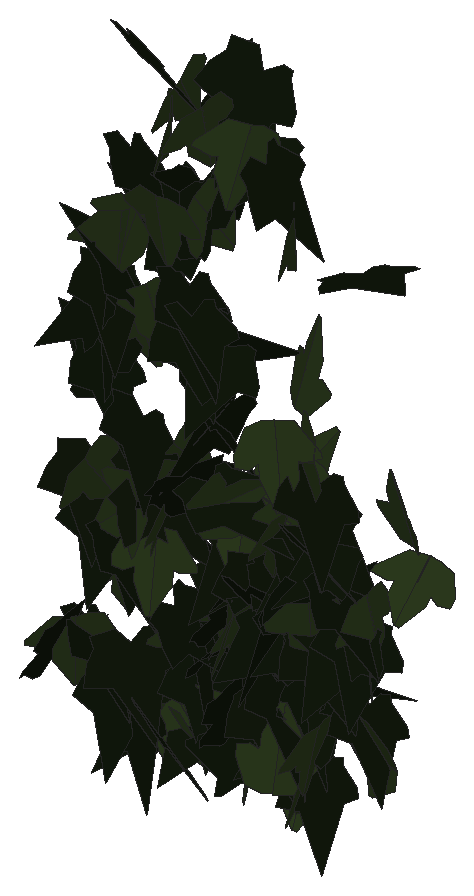
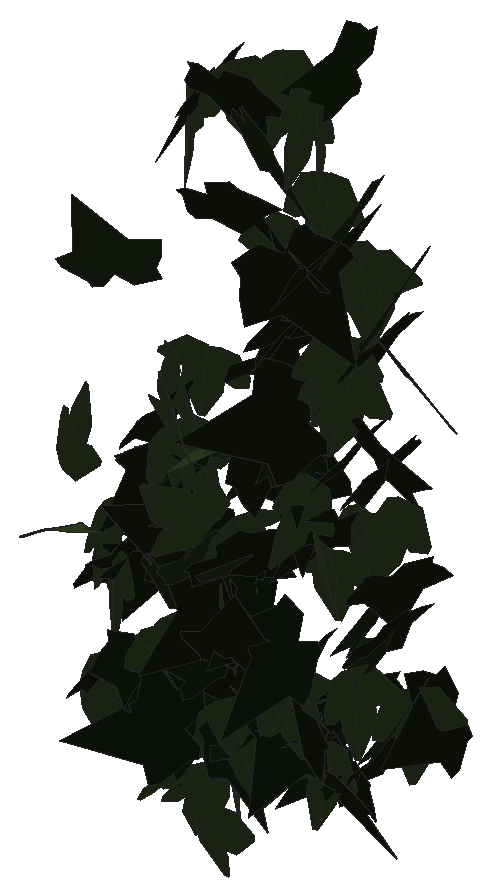
# SketchUp Ruby script. Lengths in inches.
U = 1.inch
M = Sketchup.active_model
def pt(a) = Geom::Point3d.new(a.map { |v| v * U })
def face(e, loops, mat)
  f = e.add_face(loops[0].map { |a| pt(a) })
  loops[1..].each { |l| e.add_face(l.map { |a| pt(a) }).erase! }
  f.material = f.back_material = mat if mat
  f
end
# faces: each face lists its corners as indices into pts; further lists are holes
def faces(e, pts, list, mat = nil) = list.each { |f| face(e, (f[0].is_a?(Array) ? f : [f]).map { |l| l.map { |i| pts[i] } }, mat) }
# xy, xz, yz: faces in a plane at the given z, y or x. An outline is a flat list of corners, or four numbers for a rectangle; further outlines are holes
def ring(l) = l.size == 4 ? [[l[0], l[1]], [l[2], l[1]], [l[2], l[3]], [l[0], l[3]]] : l.each_slice(2).to_a
def flat(e, list, mat, &to3) = list.each { |f| face(e, (f[0].is_a?(Array) ? f : [f]).map { |l| ring(l).map { |u, v| to3.(u, v) } }, mat) }
def xy(e, z, list, mat = nil) = flat(e, list, mat) { |x, y| [x, y, z] }
def xz(e, y, list, mat = nil) = flat(e, list, mat) { |x, z| [x, y, z] }
def yz(e, x, list, mat = nil) = flat(e, list, mat) { |y, z| [x, y, z] }
def lines(e, pts, list) = list.each { |a, b| e.add_line(pt(pts[a]), pt(pts[b])) }
# prism: a flat outline (further loops are holes) pulled along v
def prism(e, loops, v, mat = nil)
  f = face(e, loops, mat); d = Geom::Vector3d.new(v.map { |x| x * U })
  f.pushpull(f.normal.samedirection?(d) ? d.length : -d.length)
end
def box(e, o, s, mat = nil) = prism(e, [[o, [o[0] + s[0], o[1], o[2]], [o[0] + s[0], o[1] + s[1], o[2]], [o[0], o[1] + s[1], o[2]]]], [0, 0, s[2]], mat)
def at(x, y, z, deg = 0) = Geom::Transformation.translation(pt([x, y, z])) * Geom::Transformation.rotation(ORIGIN, Z_AXIS, deg.degrees)
def axes(o, x, y, z) = Geom::Transformation.new([*x, 0, *y, 0, *z, 0, *pt(o).to_a, 1])
def part(name) = M.definitions.add(name)
# library, detail: a bought-in or finely detailed component or shape, given as its bounding box
def library(name, o, s) = part(name).tap { |d| box(d.entities, o, s) }
def detail(e, o, s) = box(e.add_group.entities, o, s)
def put(e, d, t, mat = nil) = e.add_instance(d, t).tap { |i| i.material = mat if mat }
def group(e, t, mat = nil) = e.add_group.tap { |g| g.transformation = t; g.material = mat if mat }.entities
root = M.entities
M.materials.add("efeu1").color = [18, 25, 13]
M.materials.add("efeu2").color = [43, 57, 29]
c1 = part("ivyleaf_9")
p = [[1.54,2.16,1.25],[1.36,2.04,1.19],[-0.21,0.99,0.68],[-0.71,1.11,0.82],[-0.85,0.86,0.67],[-0.8,0.17,0.21],
  [-0.9,-0.01,0.1],[-0.67,-0.16,-0.02],[-0.08,-0.08,-0.05],[-0.03,-0.6,-0.4],[0.65,-0.88,-0.66],[0.83,-0.6,-0.49],
  [1.29,-0.42,-0.43],[1.8125,-0.07,-0.26],[1.21,0.44,0.15]]
faces(c1.entities,p,[[0,1,2,3,4,5,6,7,8,9,10,11,12,13,14]],"efeu1")
c2 = part("ivyleaf_10")
p = [[0,0.5,-0.03],[-0.0625,2.02,-0.43],[-0.19,2.01,-0.46],[-0.54,1.05,-0.29],[-0.52,0.625,-0.18],[-0.83,0.76,-0.28],
  [-1.16,0.64,-0.33],[-1.15,0.33,-0.24],[-0.77,-0.39,0.02],[-0.3,-0.51,0.16],[0.04,-0.48,0.23],[-0.02,2.01,-0.4375],
  [-0.06,2.01,-0.43],[0.04,-0.49,0.23],[0.67,-0.49,0.14],[1.38,0.36,-0.2],[1.375,0.51,-0.24],[0.81,0.65,-0.19],
  [0.62,0.59,-0.15],[0.6,1.09,-0.28],[0.5,1.23,-0.31]]
faces(c2.entities,p,[[0,1,2,3,4,5,6,7,8,9,10],[11,12,0,13,14,15,16,17,18,19,20]],"efeu2")
put(root,c1,axes([582.32,125.33,288.02],[0.11381,-1.15504,0.28047],[0.07251,-0.27448,-1.1598],[1.18639,0.12758,0.04398]))
put(root,c2,axes([586.27,123.92,286.54],[0.03963,-0.45785,1.13674],[0.3069,1.1048,0.43429],[-1.18643,0.27049,0.15031]))
put(root,c1,axes([581.23,125.39,277.38],[-0.01575,-1.11088,0.30737],[-0.01272,-0.30721,-1.11097],[1.15255,-0.01857,-0.00806]))
put(root,c1,axes([587.77,125.67,281.72],[-0.57329,-0.70023,0.75452],[-0.15569,-0.79473,-0.85583],[1.01754,-0.51612,0.29416]))
put(root,c1,axes([585.92,124.72,287.06],[0.58993,-1.05394,-0.28035],[0.52832,0.55501,-0.9748],[0.95408,0.34434,0.71314]))
put(root,c2,axes([583.68,124.59,296.86],[-1.21944,-0.01407,0.12592],[-0.12613,0.01907,-1.21935],[0.01203,-1.22578,-0.02042]))
put(root,c1,axes([579.36,123.72,278.95],[0.33406,0.74247,0.95484],[0.35693,0.88596,-0.81379],[-1.15567,0.48825,0.02467]))
put(root,c2,axes([588.58,124.4375,277.23],[0.7265,0.90655,-0.29073],[0.17692,0.23079,1.16172],[0.93545,-0.74771,0.00608]))
put(root,c2,axes([583.125,124.88,283.79],[1.14935,0.31036,0.07747],[0.07446,0.02141,-1.19052],[-0.31109,1.15176,0.00126]))
put(root,c2,axes([579.9,124.83,279.56],[-0.77959,-0.93319,-0.00787],[0.01313,-0.00072,-1.21594],[0.93314,-0.77963,0.01054]))
put(root,c1,axes([582.11,124.99,279.54],[-0.11229,-1.01707,-0.53891],[0.12065,0.52808,-1.02178],[1.14468,-0.15544,0.05483]))
put(root,c2,axes([589.2,124.55,298.05],[0.51429,-0.9749,-0.54171],[-0.04264,0.5789,-1.08233],[1.11448,0.47203,0.20857]))
put(root,c2,axes([582.35,124.67,285.22],[0.76174,-0.43114,-0.89495],[-0.75671,0.47882,-0.87475],[0.64359,1.07327,0.03075]))
put(root,c2,axes([586.78,125.26,300.19],[-0.84527,-0.81197,0.36804],[0.01669,-0.5215,-1.11221],[0.89133,-0.76025,0.36985]))
put(root,c1,axes([580.97,124.9375,292.34],[-1.08021,0.53868,0.08199],[-0.07975,0.0238,-1.20699],[-0.53902,-1.08306,0.01426]))
put(root,c2,axes([585.31,124.73,300.8],[-0.27892,-1.12787,-0.34975],[0.10249,0.33489,-1.1617],[1.17639,-0.29659,0.01829]))
put(root,c2,axes([589.78,125.02,278.74],[0.07235,-1.17115,-0.05305],[-0.00402,0.05291,-1.17338],[1.17235,0.07246,-0.00075]))
put(root,c1,axes([582.27,125.26,277],[-0.60107,-0.14295,-0.98246],[0.97774,0.11407,-0.61478],[0.17229,-1.14608,0.06136]))
put(root,c2,axes([586.47,124.58,282.11],[0.40839,-0.88038,-0.73105],[-0.27901,0.67618,-0.97016],[1.1098,0.49396,0.02511]))
put(root,c2,axes([588.13,124.97,289.5],[1.1256,0.39307,0.26807],[0.24844,0.10164,-1.19218],[-0.40577,1.15261,0.01371]))
put(root,c1,axes([587.93,125.68,282.8125],[-0.33573,0.20957,-1.18902],[0.85317,-0.83205,-0.38755],[-0.85427,-0.91333,0.08024]))
put(root,c1,axes([580.79,125.65,292.81],[0.09379,-1.20055,0.13025],[0.02253,-0.12888,-1.20415],[1.20739,0.09567,0.01235]))
put(root,c1,axes([588.03,124.85,299.74],[0.67435,-0.87735,-0.67896],[-0.34014,0.59278,-1.10382],[1.05596,0.75123,0.07804]))
put(root,c2,axes([580.66,124.62,286.1],[-0.22909,-0.9441,-0.70391],[0.22516,0.66876,-0.97023],[1.1559,-0.31738,0.04948]))
put(root,c1,axes([587.85,125.54,279.83],[0.34919,-1.13536,0.06954],[0.02605,-0.06474,-1.18783],[1.13719,0.35012,0.00585]))
put(root,c1,axes([582.7,125,277.22],[1.07971,-0.55791,-0.08008],[-0.07313,0.03292,-1.21533],[0.55886,1.08218,-0.00431]))
put(root,c1,axes([587.06,124.83,277.3125],[-0.73307,0.63328,0.67202],[-0.54169,0.39997,-0.96781],[-0.74782,-0.91051,0.04226]))
put(root,c2,axes([589.54,125.14,283.34],[-0.7903,-0.84131,-0.05623],[0.03542,0.04387,-1.15428],[0.84244,-0.79108,-0.00422]))
put(root,c1,axes([584.51,124.72,286.87],[0.22745,1.20382,-0.2439],[-0.07028,-0.23489,-1.22487],[-1.22627,0.23675,0.02496]))
put(root,c1,axes([586.28,124.23,278.5],[0.3056,0.48694,1.04713],[0.56521,0.8815,-0.57487],[-1.00704,0.64251,-0.00489]))
put(root,c1,axes([580.9,125.4,283.04],[0.73141,-0.91981,-0.06111],[-0.02373,0.05919,-1.17502],[0.92153,0.73157,0.01824]))
put(root,c1,axes([584.33,125.45,292.44],[0.0242,-1.10169,-0.44547],[-0.0369,0.44465,-1.10167],[1.18777,0.03626,-0.02515]))
put(root,c2,axes([583.71,124.91,300.01],[0.47808,-0.9476,-0.6718],[-0.19658,0.64999,-1.05674],[1.14482,0.50734,0.09909]))
put(root,c1,axes([581.95,125.34,302.26],[0.95204,-0.71718,0.30665],[0.3163,-0.08732,-1.18621],[0.71297,0.99639,0.11677]))
put(root,c1,axes([579.9,125.49,279.47],[0.66328,-1.02238,-0.06829],[-0.0305,0.06162,-1.21866],[1.02421,0.66393,0.00794]))
put(root,c1,axes([587.09,124.89,283.32],[1.01321,0.33232,-0.50112],[-0.48278,-0.13571,-1.06613],[-0.35843,1.12218,0.01947]))
put(root,c1,axes([589.58,125.66,277.04],[-0.68454,-0.45883,-0.79864],[0.7877,0.22408,-0.8039],[0.47737,-1.02772,0.18128]))
put(root,c2,axes([581.36,125.37,295.14],[-0.74509,-0.96458,0.06572],[-0.03238,-0.05802,-1.2188],[0.96627,-0.74573,0.00983]))
put(root,c2,axes([583.15,125.47,284.97],[0.49023,-1.07724,-0.05366],[-0.00082,0.05857,-1.18331],[1.07857,0.48966,0.02349]))
put(root,c2,axes([588.16,125.39,286.1875],[0.11049,-1.18793,-0.14228],[-0.03442,0.13967,-1.19287],[1.19592,0.11377,-0.02118]))
put(root,c2,axes([586.67,125.38,282.1875],[0.06263,-1.22048,-0.17991],[-0.02676,0.17875,-1.22197],[1.23338,0.06585,-0.01737]))
put(root,c1,axes([589.29,125.96,287.63],[0.04034,-1.20572,0.01202],[-0.01409,-0.0125,-1.2063],[1.20569,0.04019,-0.0145]))
put(root,c1,axes([580.91,125.97,293.15],[0.3457,-1.16697,0.13094],[-0.03664,0.12571,1.2171],[-1.17372,-0.34764,0.00057]))
put(root,c1,axes([586.99,125.67,279.88],[0.70848,-0.93862,0.00574],[-0.00094,-0.0079,-1.17598],[0.93863,0.70846,-0.00551]))
put(root,c1,axes([587.39,125.75,279.1],[-0.02146,-1.09655,-0.41176],[0.09209,0.40897,-1.09393],[1.16768,-0.05241,0.07871]))
put(root,c2,axes([581.88,125.58,295.42],[-1.10791,-0.23795,0.45365],[-0.41085,-0.2329,-1.12554],[0.30598,-1.17432,0.13131]))
put(root,c1,axes([585.02,126.34,291.18],[-0.52681,-1.03663,0.25903],[0.01019,-0.29367,-1.1545],[1.06845,-0.50832,0.13873]))
put(root,c1,axes([582.64,125.33,285.59],[0.23735,-0.79333,-0.84105],[0.14695,0.87233,-0.78136],[1.1468,0.05242,0.27419]))
put(root,c1,axes([589.85,126.04,285.625],[-1.14365,-0.31881,0.16691],[-0.16527,-0.02864,-1.18714],[0.31966,-1.15541,-0.01662]))
put(root,c1,axes([588.92,126.18,278.83],[-1.08156,-0.38687,0.23688],[-0.17328,-0.21366,-1.14012],[0.41923,-1.08639,0.13988]))
put(root,c1,axes([590.37,126.22,282.46],[-0.7341,-0.9033,0.06874],[-0.04584,-0.05132,-1.16398],[0.90475,-0.73553,-0.0032]))
put(root,c2,axes([588.59,125.99,286.72],[-0.46943,-1.05431,0.34154],[-0.00233,-0.36998,-1.14529],[1.10825,-0.44736,0.14226]))
put(root,c1,axes([586.52,126.22,283.18],[-0.01509,-1.14507,0.06503],[0.01509,-0.06523,-1.14506],[1.14681,-0.01421,0.01592]))
put(root,c1,axes([584.73,124.96,288.09],[-0.21261,1.17745,0.41264],[-0.10765,0.39972,-1.19603],[-1.24301,-0.23601,0.033]))
put(root,c1,axes([588.71,125.05,282.54],[0.06156,-0.05828,1.23131],[1.06825,0.61772,-0.02417],[-0.61511,1.06694,0.08125]))
put(root,c2,axes([582.81,125.62,277.01],[-1.13672,0.1388,0.06251],[-0.06298,-0.00011,-1.14513],[-0.13859,-1.13843,0.00773]))
put(root,c1,axes([588.13,126,285.57],[0.77889,-0.74968,0.40969],[0.41007,-0.15829,-1.06926],[0.74948,0.86571,0.15927]))
put(root,c1,axes([581.28,126.1,297.47],[0.6991,-1.07923,-0.03858],[-0.01931,0.03346,-1.28587],[1.07974,0.69936,0.00198]))
put(root,c1,axes([589.49,125.98,282.11],[-0.11503,-0.99117,-0.6294],[0.18516,0.60919,-0.99318],[1.15943,-0.19562,0.09617]))
put(root,c2,axes([589.3,125.49,288.79],[-0.35489,0.28503,1.11686],[-1.0918,0.29158,-0.42134],[-0.3696,-1.13504,0.17223]))
put(root,c1,axes([589.83,125.95,284.07],[0.63064,-0.9662,-0.27803],[-0.08448,0.27612,-1.15116],[1.00185,0.63148,0.07794]))
put(root,c1,axes([579.89,126.64,282.97],[-0.22103,-1.12341,0.28174],[0.01153,-0.28894,-1.1431],[1.15815,-0.21153,0.06515]))
put(root,c1,axes([583.54,126.35,292.92],[0.41384,-1.26878,-0.00115],[-0.00114,0.00083,-1.33457],[1.26878,0.41384,-0.00082]))
put(root,c1,axes([579.5625,126.32,285.07],[-0.34812,-1.09279,-0.28599],[0.07094,0.27752,-1.14678],[1.12736,-0.35491,-0.01615]))
put(root,c2,axes([588.78,125.69,276.59],[0.32901,-0.90558,-0.61868],[-0.16106,0.59902,-0.96246],[1.08485,0.36358,0.04474]))
put(root,c1,axes([583.97,126.83,277.08],[-0.56345,-0.92631,0.35645],[-0.12055,-0.34298,-1.08186],[0.98518,-0.57175,0.07148]))
put(root,c1,axes([581.98,126.39,276.81],[-1.15193,0.12858,-0.12998],[0.13116,0.00352,-1.15895],[-0.12737,-1.15924,-0.01793]))
put(root,c1,axes([590.56,126.75,282.21],[-0.24052,-1.13583,0.03593],[-0.00506,-0.03565,-1.16101],[1.13638,-0.24056,0.00243]))
put(root,c2,axes([585.41,126.8125,285.03],[-0.63649,-0.92542,0.48586],[0.53729,-0.77763,-0.7773],[0.89654,-0.19097,0.81076]))
put(root,c1,axes([579.8,126.58,289.07],[0.24732,-1.16077,-0.07889],[-0.00565,0.07946,-1.18678],[1.16344,0.24714,0.01101]))
put(root,c1,axes([580.3,126.98,281.6],[0.08473,-0.87773,0.74277],[0.30345,-0.70131,-0.86335],[1.10907,0.25894,0.17947]))
put(root,c2,axes([583.73,125.81,277.23],[0.52789,0.94038,0.57255],[0.28984,0.49386,-1.07837],[-1.06213,0.60215,-0.00971]))
put(root,c2,axes([581.97,126.16,292.27],[-0.68604,-0.93093,-0.32293],[0.3021,0.17582,-1.14865],[0.9379,-0.73758,0.13377]))
put(root,c1,axes([588.92,125.85,285.95],[0.0668,-0.52458,-1.08541],[0.05671,1.08724,-0.52197],[1.20419,-0.0221,0.08479]))
put(root,c1,axes([583.24,126.01,280.91],[0.66171,-0.69093,-0.69381],[-0.25742,0.68518,-0.92784],[0.94472,0.67065,0.23315]))
put(root,c1,axes([585.32,125.33,281.59],[0.35868,0.84748,0.81551],[0.29581,0.76017,-0.92009],[-1.13832,0.46458,0.01786]))
put(root,c1,axes([585.79,127.27,284.06],[-0.74999,-1.02032,0.45254],[-0.27483,-0.35962,-1.26628],[1.08181,-0.79872,-0.00796]))
put(root,c1,axes([584.54,127.23,288.58],[-0.4256,0.14484,-1.23062],[0.63691,-1.09057,-0.34862],[-1.0629,-0.71148,0.28385]))
put(root,c2,axes([586.09,126.48,276.55],[0.69426,-0.92357,-0.08588],[0.01125,0.11565,-1.15276],[0.92749,0.68993,0.07827]))
put(root,c1,axes([588.37,126.87,279.2],[0.20678,-1.13343,-0.00739],[-0.02817,0.00237,-1.15182],[1.13311,0.2069,-0.02729]))
put(root,c2,axes([581.42,126.31,291.45],[-1.12162,-0.3878,-0.16179],[0.14239,0.0831,-1.18634],[0.39533,-1.13017,-0.03172]))
put(root,c1,axes([586.66,127.42,283.28],[-0.62926,-0.91583,0.47867],[0.53116,-0.76739,-0.76995],[0.88642,-0.1903,0.80118]))
put(root,c1,axes([583.89,127,278.33],[-0.17257,-1.1516,-0.10953],[-0.00733,0.11183,-1.16422],[1.15677,-0.17109,-0.02372]))
put(root,c2,axes([590.86,126.52,283.4],[-0.01384,-1.14695,-0.22001],[0.31095,0.20846,-1.10632],[1.1257,-0.07169,0.3029]))
put(root,c2,axes([583.37,126.86,279.78],[-0.49057,-1.02197,0.2909],[-0.0178,-0.31246,-1.12773],[1.06242,-0.47713,0.11543]))
put(root,c2,axes([583.32,126.16,300.68],[-0.06021,-1.03209,-0.70247],[0.01091,0.70282,-1.03355],[1.24842,-0.05592,-0.02485]))
put(root,c1,axes([580.38,126.08,289],[-0.25644,0.53419,1.15943],[-0.845,0.8154,-0.56258],[-0.95687,-0.86323,0.18608]))
put(root,c2,axes([586.02,126.65,282.09],[0.43547,-1.08578,-0.13815],[0.00771,0.15172,-1.16815],[1.09451,0.43093,0.06319]))
put(root,c1,axes([582.81,126.91,279.33],[-0.36514,-0.16626,-1.26907],[1.24412,0.26378,-0.39252],[0.30054,-1.29394,0.08305]))
put(root,c1,axes([582.6875,127.36,294.59],[-0.12577,-1.37324,-0.16711],[0.15663,-0.18086,1.36832],[-1.37448,0.10505,0.17122]))
put(root,c1,axes([583.53,126.53,289.17],[1.12955,-0.65274,-0.22215],[-0.18062,0.13137,-1.30439],[0.66543,1.14367,0.02303]))
put(root,c2,axes([587.44,127.61,286.77],[-0.89998,-0.45285,0.69145],[0.54805,-1.09214,-0.00195],[0.61873,0.30868,1.00749]))
put(root,c1,axes([585.71,127.3,301.4],[-1.21078,-0.48911,-0.46539],[0.44661,0.13639,-1.30528],[0.50632,-1.28995,0.03845]))
put(root,c2,axes([590.58,126.55,281.7],[0.89829,-0.61811,-0.43066],[-0.08572,0.58198,-1.0141],[0.74845,0.80851,0.40073]))
put(root,c1,axes([588.68,126.93,282.375],[-0.97778,0.60106,-0.12432],[0.0955,-0.08201,-1.14759],[-0.60631,-0.98224,0.01974]))
put(root,c2,axes([583.07,126.34,286.79],[-0.21386,-0.89408,-0.81791],[0.25413,0.77898,-0.91798],[1.1848,-0.32847,0.04926]))
put(root,c2,axes([587.37,127.73,275.69],[-0.86033,-0.66411,0.44976],[0.52528,-0.96495,-0.42004],[0.60614,-0.10638,1.00238]))
put(root,c1,axes([588.36,127,279.21],[-0.9641,0.6224,0.12997],[-0.10607,0.07532,-1.14753],[-0.62691,-0.9699,-0.00572]))
put(root,c1,axes([584.11,126.61,295.39],[-0.38078,0.51065,1.04767],[-0.74085,0.74479,-0.63229],[-0.89973,-0.82939,0.07725]))
put(root,c1,axes([590.13,127.54,278.88],[0.12493,-1.14106,-0.07944],[0.0174,0.0818,-1.14758],[1.14369,0.1234,0.02613]))
put(root,c1,axes([585.79,126.21,277.66],[0.38063,0.71752,0.80645],[-0.23531,0.88971,-0.68054],[-1.05349,0.06051,0.44338]))
put(root,c1,axes([586.45,126.89,280.18],[0.99086,-0.36703,0.46081],[0.54368,0.22244,-0.99187],[0.22688,1.0699,0.3643]))
put(root,c1,axes([583.49,126.25,278.3],[0.40047,1.10053,0.49648],[0.11296,0.48663,-1.16981],[-1.20203,0.41238,0.05548]))
put(root,c2,axes([583.95,126.53,296.07],[0.0796,0.96536,0.75805],[-0.22017,0.75855,-0.94288],[-1.20751,-0.07467,0.22189]))
put(root,c2,axes([580.29,127.38,281.29],[-0.31744,-1.10789,-0.0389],[0.00287,0.03964,-1.15245],[1.10857,-0.31735,-0.00815]))
put(root,c2,axes([587.83,127.35,280.19],[-0.97332,-0.61456,-0.04753],[0.02548,0.04865,-1.15078],[0.61587,-0.97327,-0.02751]))
put(root,c2,axes([590.99,127.11,277.37],[-0.07808,0.19579,-1.25186],[-1.07361,0.6559,0.16955],[0.67295,1.06913,0.12524]))
put(root,c1,axes([582.79,127.64,296.14],[0.04399,0.9103,-1.04571],[-0.56063,-0.9452,-0.84639],[-1.26801,0.44948,0.33794]))
put(root,c2,axes([591.6,127.625,286.04],[-1.06089,0.52073,-0.11674],[-0.10074,0.05968,1.18176],[0.52406,1.06562,-0.00914]))
put(root,c1,axes([584.33,127.66,300.33],[-1.11893,0.7619,-0.11152],[0.09897,-0.05279,-1.35365],[-0.76363,-1.12324,-0.01203]))
put(root,c1,axes([585.81,126.98,281.95],[0.91155,0.58087,0.43213],[0.3854,0.19885,-1.08027],[-0.61287,0.989,-0.0366]))
put(root,c2,axes([584.82,127.88,278.8],[-1.02673,-0.57151,0.44212],[-0.37511,-0.235,-1.17488],[0.61756,-1.0929,0.02143]))
put(root,c1,axes([585.21,127.76,277.95],[-0.59455,0.93192,-0.26403],[0.11863,-0.23741,-1.1051],[-0.96131,-0.60567,0.02692]))
put(root,c1,axes([587.4,127.3,278.48],[0.19614,1.12783,0.06991],[-0.31327,0.12245,-1.09646],[-1.0857,0.16842,0.32901]))
put(root,c1,axes([582.48,127.26,290.11],[0.91407,0.29831,1.00805],[0.96275,0.29896,-0.96146],[-0.42221,1.32752,-0.00999]))
put(root,c1,axes([588.82,127.41,279.42],[0.11922,1.14054,0.05735],[-0.12643,0.07049,-1.13903],[-1.13496,0.11195,0.1329]))
put(root,c2,axes([591.25,128.98,283.83],[-1.08793,-0.33795,0.2691],[0.30476,-1.11719,-0.17092],[0.30618,-0.08879,1.12631]))
put(root,c1,axes([584.98,128.71,298.0625],[-1.24929,-0.47857,0.03569],[-0.0303,-0.02068,-1.33779],[0.47894,-1.24963,0.00847]))
put(root,c1,axes([584.8,127.94,281.15],[-1.17178,-0.20254,0.40296],[0.39704,0.06881,1.18916],[-0.21391,1.23722,-0.00017]))
put(root,c1,axes([582.3125,127.88,282.39],[1.35604,0.02886,-0.24012],[-0.24041,0.01226,-1.35624],[-0.02628,1.37708,0.01711]))
put(root,c2,axes([585.55,128.19,276.73],[0.21933,1.19594,0.05249],[0.00776,0.05195,-1.21588],[-1.19706,0.21946,0.00173]))
put(root,c1,axes([588.75,128.98,294.2],[0.03098,-1.18389,0.25325],[1.14902,-0.05106,-0.37925],[0.38141,0.24998,1.12193]))
put(root,c2,axes([586.07,128.02,285.67],[0.53242,0.58045,-0.99297],[0.67944,0.72416,0.78762],[0.92805,-0.86317,-0.00696]))
put(root,c2,axes([586.24,128.88,289.02],[1.09051,-0.63691,0.02862],[0.002,0.06013,1.26178],[-0.63755,-1.08923,0.05292]))
put(root,c1,axes([586.27,128.75,278.31],[1.08908,-0.16227,0.75228],[0.76906,0.27775,-1.05345],[-0.0285,1.29417,0.32042]))
put(root,c2,axes([584.77,129.07,275.66],[-0.16539,0.10627,-1.25252],[-1.06837,0.65377,0.19654],[0.66234,1.08108,0.00427]))
